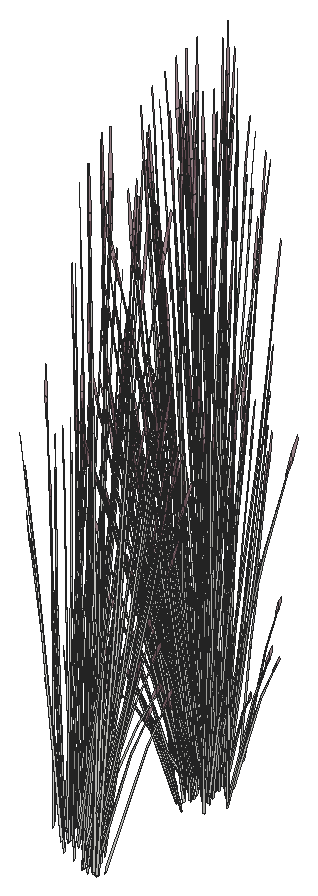
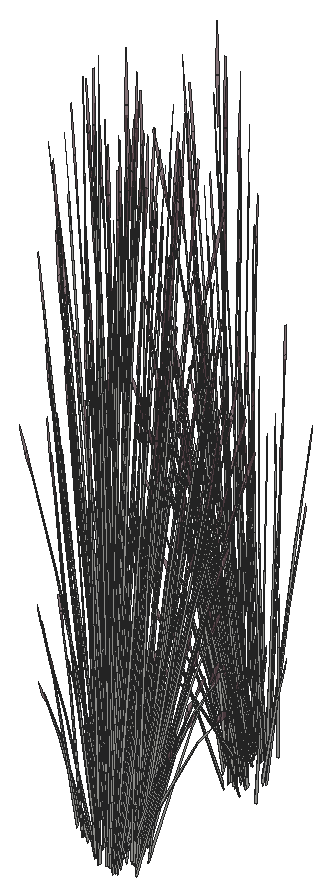
# SketchUp Ruby script. Lengths in inches.
U = 1.inch
M = Sketchup.active_model
def pt(a) = Geom::Point3d.new(a.map { |v| v * U })
def face(e, loops, mat)
  f = e.add_face(loops[0].map { |a| pt(a) })
  loops[1..].each { |l| e.add_face(l.map { |a| pt(a) }).erase! }
  f.material = f.back_material = mat if mat
  f
end
# faces: each face lists its corners as indices into pts; further lists are holes
def faces(e, pts, list, mat = nil) = list.each { |f| face(e, (f[0].is_a?(Array) ? f : [f]).map { |l| l.map { |i| pts[i] } }, mat) }
# xy, xz, yz: faces in a plane at the given z, y or x. An outline is a flat list of corners, or four numbers for a rectangle; further outlines are holes
def ring(l) = l.size == 4 ? [[l[0], l[1]], [l[2], l[1]], [l[2], l[3]], [l[0], l[3]]] : l.each_slice(2).to_a
def flat(e, list, mat, &to3) = list.each { |f| face(e, (f[0].is_a?(Array) ? f : [f]).map { |l| ring(l).map { |u, v| to3.(u, v) } }, mat) }
def xy(e, z, list, mat = nil) = flat(e, list, mat) { |x, y| [x, y, z] }
def xz(e, y, list, mat = nil) = flat(e, list, mat) { |x, z| [x, y, z] }
def yz(e, x, list, mat = nil) = flat(e, list, mat) { |y, z| [x, y, z] }
def lines(e, pts, list) = list.each { |a, b| e.add_line(pt(pts[a]), pt(pts[b])) }
# prism: a flat outline (further loops are holes) pulled along v
def prism(e, loops, v, mat = nil)
  f = face(e, loops, mat); d = Geom::Vector3d.new(v.map { |x| x * U })
  f.pushpull(f.normal.samedirection?(d) ? d.length : -d.length)
end
def box(e, o, s, mat = nil) = prism(e, [[o, [o[0] + s[0], o[1], o[2]], [o[0] + s[0], o[1] + s[1], o[2]], [o[0], o[1] + s[1], o[2]]]], [0, 0, s[2]], mat)
def at(x, y, z, deg = 0) = Geom::Transformation.translation(pt([x, y, z])) * Geom::Transformation.rotation(ORIGIN, Z_AXIS, deg.degrees)
def axes(o, x, y, z) = Geom::Transformation.new([*x, 0, *y, 0, *z, 0, *pt(o).to_a, 1])
def part(name) = M.definitions.add(name)
# library, detail: a bought-in or finely detailed component or shape, given as its bounding box
def library(name, o, s) = part(name).tap { |d| box(d.entities, o, s) }
def detail(e, o, s) = box(e.add_group.entities, o, s)
def put(e, d, t, mat = nil) = e.add_instance(d, t).tap { |i| i.material = mat if mat }
def group(e, t, mat = nil) = e.add_group.tap { |g| g.transformation = t; g.material = mat if mat }.entities
root = M.entities
M.materials.add("LightPink_Translucent").color = [144, 107, 117]
M.materials["LightPink_Translucent"].alpha = 0.75
c1 = part("blade")
p = [[2.15,0.21,22],[0,0.17,0],[0.09,0.45,0],[2.18,0.31,22],[2.29,0.31,22],[0.38,0.45,0],
  [2.48,0.24,33],[2.49,0.24,33],[2.48,0.22,33]]
faces(c1.entities,p,[[0,1,2,3],[4,5,2,3],[6,3,4,7],[8,0,3,6]])
c2 = part("seeds")
p = [[0.3,-0.1,1.38],[-0.01,-0.03,1.59],[-0.01,-0.03,0.03],[0.14,-0.07,-0.07],[0.29,-0.03,3],[0.15,0.01,3.11]]
faces(c2.entities,p,[[0,1,2,3],[1,0,4,5]],"LightPink_Translucent")
c3 = part("blade with seeds")
put(c3.entities,c1,at(0,0,0))
put(c3.entities,c2,axes([2.4,0.25,30.99],[1.5799,-0.05474,1.17369],[-0.12525,1.92788,0.29478],[-0.07173,-0.02425,1.56792]))
put(root,c3,axes([331.53,378.59,1400.62],[0.26075,0.2802,0.1448],[-0.2175,0.31612,-0.41347],[-0.06054,0.04274,1.26744]))
put(root,c3,axes([329.47,378.67,1402.73],[-0.08753,-0.42921,0.48003],[0.34336,-0.07449,0.3958],[-0.1012,0.10094,0.9933]))
put(root,c3,axes([329.41,378.58,1402.73],[-0.2423,-0.19613,0.0643],[0.14107,-0.2793,0.50621],[-0.07768,0.0903,0.77189]))
put(root,c3,axes([329.52,378.07,1401.875],[0.12246,-0.09864,1.71376],[0.1031,0.45582,0.13857],[-0.19225,0.10302,0.73262]))
put(root,c3,axes([332.21,379.08,1402.98],[0.35281,0.01123,-0.71045],[-0.0237,0.47284,0.08574],[0.14947,0.0499,1.00501]))
put(root,c3,axes([331.8125,379.46,1400.48],[0.33032,-0.23318,0.49651],[0.19744,0.41812,0],[-0.07523,0.05311,1.57504]))
put(root,c3,axes([331.34,379.09,1400.29],[0.15345,0.53576,-0.06012],[-0.43845,0.18773,0],[0.00536,0.01871,1.72173]))
put(root,c3,axes([331.51,379.67,1400.03],[-0.32928,-0.11539,-0.30978],[0.08291,-0.40636,0.30978],[-0.06638,0.04686,1.38974]))
put(root,c3,axes([329.14,378.84,1400.59],[0.12266,0.03828,1.43002],[0.07906,0.39104,-0.30754],[-0.16661,0.0732,0.61141]))
put(root,c3,axes([329.6875,378.52,1403.05],[0.30722,-0.06665,0.35414],[0.08112,0.381,-0.4572],[-0.08804,0.10234,0.87481]))
put(root,c3,axes([332.78,378.12,1400.375],[0.44133,0,0],[0,0.52122,-0.51607],[0,0.11871,1.63711]))
put(root,c3,axes([328.5,378.35,1402.71],[0.04504,0.01251,1.77383],[0.13934,0.41205,-0.16761],[-0.0922,0.10815,0.31391]))
put(root,c3,axes([332.61,378.38,1400.2],[-0.44111,-0.00373,-0.04976],[0,-0.52122,0.49943],[-0.01386,0.11865,1.58352]))
put(root,c3,axes([331.65,377.93,1400.67],[0.39748,0.22252,-0.29095],[-0.19139,0.46966,-0.50002],[0.01249,0.11531,1.59708]))
put(root,c3,axes([328.88,379.66,1400.77],[0.14709,-0.21136,1.1486],[0.05804,0.3346,0.84392],[-0.1063,0.05991,0.25299]))
put(root,c3,axes([332.42,379.27,1402.53],[0.20082,0.29199,-0.35414],[-0.2293,0.2764,0.4572],[0.1165,0.04206,0.87481]))
put(root,c3,axes([332.52,378.46,1400.03],[-0.24637,0.29097,-0.30978],[-0.24637,-0.29097,0.30978],[0,0.09372,1.38974]))
put(root,c3,axes([331.46,378.49,1400.67],[0.04113,0.53214,-0.29095],[-0.42835,0.03218,-0.50002],[-0.07543,0.07088,1.59708]))
put(root,c3,axes([332.32,379.38,1402.73],[-0.01777,0.35463,0.0643],[-0.26836,-0.00972,0.50621],[0.1028,0.03711,0.77189]))
put(root,c3,axes([331.61,378.28,1400.21],[-0.17124,0.42022,-0.44739],[-0.35581,-0.20224,0.21531],[0,0.09687,1.43643]))
put(root,c3,axes([329.43,378.75,1402.53],[-0.30722,0.06665,-0.35414],[-0.08112,-0.381,0.4572],[-0.08804,0.10234,0.87481]))
put(root,c3,axes([332.34,379.27,1402.73],[-0.26024,0.30729,0.48003],[-0.22444,-0.32634,0.3958],[0.1221,0.05668,0.9933]))
put(root,c3,axes([328.99,379.6,1403.65],[0.31145,0.12449,-0.06488],[-0.0958,0.38314,-0.29416],[-0.05094,0.05817,0.97024]))
put(root,c3,axes([331.2,378.9,1400.06],[-0.23773,0.35053,-0.62353],[-0.29532,-0.31785,-0.16365],[-0.09526,0.08744,1.37633]))
put(root,c3,axes([331.52,379.625,1403.05],[-0.05451,-0.37564,0.35414],[0.31161,-0.09919,-0.4572],[0.0837,0.10765,0.87481]))
put(root,c3,axes([331.62,379.49,1400.33],[0.44186,0.15158,0.30756],[-0.11054,0.54181,-0.36492],[-0.07313,0.06781,1.64885]))
put(root,c3,axes([331.59,379.85,1400.02],[-0.33032,0.23318,-0.49651],[-0.19744,-0.41812,0],[-0.07523,0.05311,1.57504]))
put(root,c3,axes([332.6875,378.47,1400.02],[0,0.46636,-0.49651],[-0.39487,0,0],[0,0.10622,1.57504]))
put(root,c3,axes([331.7,378.52,1401.875],[-0.1311,-0.08035,1.71376],[0.27131,-0.33708,0.13857],[0.16909,0.15206,0.73262]))
put(root,c3,axes([331.72,377.47,1402.47],[-0.30498,-0.24231,1.38283],[0.32203,-0.37727,0.59665],[0.0984,0.22736,1.33663]))
put(root,c3,axes([329.53,378.49,1403.03],[0.32648,0.25715,-0.1216],[-0.18809,0.3724,-0.67495],[-0.09224,0.12945,1.02557]))
put(root,c3,axes([332.18,379.4375,1400.77],[-0.19872,-0.13409,1.1486],[0.2566,-0.13625,0.84392],[0.06921,0.11541,0.25299]))
put(root,c3,axes([331.49,379.82,1403.03],[0.21031,-0.39918,-0.1216],[0.30457,0.22997,-0.67495],[0.10587,0.11278,1.02557]))
put(root,c3,axes([329.97,378.375,1401.875],[0.08815,-0.14329,1.71376],[0.22258,0.38678,0.13857],[-0.15267,0.17614,0.73262]))
put(root,c3,axes([329.6875,378.79,1402.68],[0.09067,0.42583,-0.51099],[-0.34336,0.07449,-0.3958],[-0.0984,0.11438,0.97773]))
put(root,c3,axes([330.1,379.28,1403.05],[0.23881,-0.24554,0.35414],[0.22606,0.28036,-0.4572],[-0.0344,0.14245,0.87481]))
put(root,c3,axes([331.89,379.78,1400.375],[0.22066,0.46731,0],[-0.36918,0.26061,-0.51607],[-0.08408,0.05936,1.63711]))
put(root,c3,axes([331.21,380.15,1402.71],[0.00104,-0.05646,1.77383],[0.30246,-0.2491,-0.16761],[0.10506,0.08891,0.31391]))
put(root,c3,axes([332.24,379.9375,1399.49],[0.02571,-0.06733,1.76342],[0.32373,-0.19829,-0.26939],[0.09815,0.10263,0.30037]))
put(root,c3,axes([331.7,377.93,1400.84],[-0.00964,-0.43909,1.41272],[0.43635,0.11382,0.59816],[-0.1032,0.24027,1.3335]))
put(root,c3,axes([331.8125,378.41,1400.09],[0.12941,0.42699,-0.69212],[-0.37279,0.15378,-0.18165],[0.0143,0.14459,1.52773]))
put(root,c3,axes([329.88,379.5,1402.73],[-0.29004,-0.02173,0.0643],[0.00795,-0.32812,0.50621],[-0.03035,0.12569,0.77189]))
put(root,c3,axes([329.27,379.88,1399.49],[0.04734,0.04659,1.76342],[0.08027,0.4317,-0.26939],[-0.10492,0.09206,0.30037]))
put(root,c3,axes([329.98,379.53,1402.73],[-0.25132,-0.3182,0.48003],[0.2669,-0.27442,0.3958],[-0.04636,0.14929,0.9933]))
put(root,c3,axes([331.74,379.62,1402.68],[0.34827,-0.11086,-0.51099],[0.06092,0.41983,-0.3958],[0.09354,0.12031,0.97773]))
put(root,c3,axes([330.77,379.6875,1403.05],[0.1064,-0.35863,0.35414],[0.31043,0.1046,-0.4572],[0.02846,0.14439,0.87481]))
put(root,c3,axes([332.22,380.05,1400.67],[-0.22633,-0.01463,1.0506],[0.14947,-0.31064,0.58006],[0.08941,0.11036,0.8241]))
put(root,c3,axes([331.56,379.97,1402.73],[-0.16041,0.29625,0.0643],[-0.22843,-0.17248,0.50621],[0.07385,0.09498,0.77189]))
put(root,c3,axes([331.1875,380.97,1403.65],[0.2439,-0.26754,-0.06488],[0.22348,0.29302,-0.29416],[0.01573,0.08303,0.97024]))
put(root,c3,axes([331.63,379.88,1402.73],[-0.35104,0.10702,0.48003],[-0.06092,-0.41983,0.3958],[0.08256,0.12373,0.9933]))
put(root,c3,axes([329.9,378.73,1401.875],[0.06572,-0.16029,1.71376],[0.27569,0.33172,0.13857],[-0.12437,0.20675,0.73262]))
put(root,c3,axes([331.48,379.3,1400.59],[0.00623,-0.15459,1.43002],[0.29764,-0.17268,-0.30754],[0.09188,0.18503,0.61141]))
put(root,c3,axes([330.67,380.01,1402.73],[-0.26007,0.1585,0.0643],[-0.12729,-0.28902,0.50621],[0.02512,0.1274,0.77189]))
put(root,c3,axes([329.98,379.63,1402.53],[-0.23881,0.24554,-0.35414],[-0.22606,-0.28036,0.4572],[-0.0344,0.14245,0.87481]))
put(root,c3,axes([329.15,379.56,1402.72],[-0.00877,0.09229,1.74944],[0.24897,0.32105,-0.27667],[-0.06518,0.15182,0.14031]))
put(root,c3,axes([329.95,379.35,1403.4],[0.3879,0.02311,-0.13498],[-0.0106,0.43749,-0.74919],[-0.02694,0.1685,1.13838]))
put(root,c3,axes([330.67,379.84,1403.03],[0.34538,-0.21713,-0.1216],[0.16972,0.38536,-0.67495],[0.04557,0.16239,1.02557]))
put(root,c3,axes([330.77,379.98,1403.0625],[-0.34777,-0.12192,0.53283],[0.11892,-0.40083,0.43934],[0.0209,0.15763,1.10256]))
put(root,c3,axes([330.13,380.58,1400.77],[-0.00913,-0.2773,1.1486],[0.22824,0.19778,0.84392],[-0.04489,0.13217,0.25299]))
put(root,c3,axes([330.73,379.92,1399.49],[0.05712,-0.02538,1.76342],[0.34359,0.13968,-0.26939],[0.01005,0.15742,0.30037]))
put(root,c3,axes([330.21,379.51,1403],[0.25266,0.31335,-0.5672],[-0.2669,0.27442,-0.43934],[-0.03844,0.15921,1.08528]))
put(root,c3,axes([329.9375,379.98,1400.82],[0.32063,-0.08258,0.06507],[0.07371,0.33271,-0.86304],[-0.02033,0.16842,0.7736]))
put(root,c3,axes([330.96,379.82,1402.68],[0.34695,0.11691,-0.51099],[-0.11892,0.40083,-0.3958],[0.03181,0.16138,0.97773]))
put(root,c3,axes([331.16,378.99,1401.875],[-0.08068,-0.14973,1.71376],[0.3728,-0.12606,0.13857],[0.08426,0.23506,0.73262]))
put(root,c3,axes([330.8,380.0625,1402.53],[-0.1064,0.35863,-0.35414],[-0.31043,-0.1046,0.4572],[0.02846,0.14439,0.87481]))
put(root,c3,axes([330.13,379.37,1403.34],[-0.00918,0.43138,-0.7886],[-0.38672,-0.02897,0.09517],[-0.04081,0.18275,1.11556]))
put(root,c3,axes([329.125,380.5,1402.71],[0.04004,-0.02816,1.77383],[0.33095,0.18728,-0.16761],[-0.00778,0.15594,0.31391]))
put(root,c3,axes([330.5,379.06,1401.875],[-0.00864,-0.17899,1.71376],[0.37441,0.11874,0.13857],[-0.02316,0.25508,0.73262]))
put(root,c3,axes([330.84,379.74,1402.98],[0.16845,0.3792,-0.71045],[-0.34676,0.21133,0.08574],[0.03939,0.18322,1.00501]))
put(root,c3,axes([329.86,380.34,1400.59],[0.11138,-0.07357,1.43002],[0.27499,0.22183,-0.30754],[-0.08185,0.19194,0.61141]))
put(root,c3,axes([330.58,380.7,1402.72],[0.04474,0.0751,1.74944],[0.36104,0.0295,-0.27667],[0.03631,0.16562,0.14031]))
put(root,c3,axes([330.01,379.98,1401.36],[0.00775,-0.24075,1.54345],[0.34877,0.12716,0.21329],[-0.03022,0.25658,0.72882]))
put(root,c3,axes([330.27,391.54,1401.875],[0.08068,0.14973,1.71376],[-0.3728,0.12606,0.13857],[-0.08426,-0.23506,0.73262]))
put(root,c3,axes([330.89,390.55,1402.72],[-0.05398,-0.06539,1.74944],[-0.36026,0.04145,-0.27667],[-0.0575,-0.15639,0.14031]))
put(root,c3,axes([331.72,391.33,1400.59],[-0.10032,0.0944,1.43002],[-0.30046,-0.16522,-0.30754],[0.05569,-0.20547,0.61141]))
put(root,c3,axes([331.27,391.66,1402.98],[-0.16845,-0.3792,-0.71045],[0.34676,-0.21133,0.08574],[-0.03939,-0.18322,1.00501]))
put(root,c3,axes([330.17,391.15,1400.59],[-0.02137,0.15256,1.43002],[-0.31245,0.12771,-0.30754],[-0.07303,-0.19719,0.61141]))
put(root,c3,axes([330.98,390.81,1399.49],[-0.0592,0.0168,1.76342],[-0.32738,-0.18913,-0.26939],[0.00549,-0.15776,0.30037]))
put(root,c3,axes([331.97,392.03,1402.98],[0.00918,-0.43138,-0.71045],[0.38672,0.02897,0.08574],[0.04081,-0.18275,1.00501]))
put(root,c3,axes([332.51,391.35,1402.72],[-0.00341,-0.09282,1.74944],[-0.28775,-0.26825,-0.27667],[0.04449,-0.16261,0.14031]))
put(root,c3,axes([331.3,391.33,1402.53],[0.1064,-0.35863,-0.35414],[0.31043,0.1046,0.4572],[-0.02846,-0.14439,0.87481]))
put(root,c3,axes([331.53,391.81,1401.875],[-0.06572,0.16029,1.71376],[-0.27569,-0.33172,0.13857],[0.12437,-0.20675,0.73262]))
put(root,c3,axes([332.43,391.02,1402.71],[-0.03584,0.03562,1.77383],[-0.35118,-0.12018,-0.16761],[-0.01271,-0.15545,0.31391]))
put(root,c3,axes([331.14,391.58,1402.68],[-0.34695,-0.11691,-0.51099],[0.11892,-0.40083,-0.3958],[-0.03181,-0.16138,0.97773]))
put(root,c3,axes([331.35,390.58,1400.77],[0.04528,0.27194,1.1486],[-0.25117,-0.15062,0.84392],[0.02703,-0.13924,0.25299]))
put(root,c3,axes([331.89,391.88,1402.68],[-0.25266,-0.31335,-0.51099],[0.2669,-0.27442,-0.3958],[0.03844,-0.15921,0.97773]))
put(root,c3,axes([330.52,390.34,1402.71],[-0.00658,0.0559,1.77383],[-0.32474,0.20287,-0.16761],[-0.09556,-0.1037,0.31391]))
put(root,c3,axes([330.45,391.33,1403.09],[0.39316,-0.11987,0.53763],[0.06823,0.47021,0.4433],[-0.09247,-0.13858,1.11249]))
put(root,c3,axes([331.34,391.42,1402.73],[0.34777,0.12192,0.48003],[-0.11892,0.40083,0.3958],[-0.0209,-0.15763,0.9933]))
put(root,c3,axes([331.4375,391.5625,1403.03],[-0.34538,0.21713,-0.1216],[-0.16972,-0.38536,-0.67495],[-0.04557,-0.16239,1.02557]))
put(root,c3,axes([332.15,392.05,1403.03],[-0.3879,-0.02311,-0.1216],[0.0106,-0.43749,-0.67495],[0.02694,-0.1685,1.02557]))
put(root,c3,axes([332.13,391.77,1402.53],[0.23881,-0.24554,-0.35414],[0.22606,0.28036,0.4572],[0.0344,-0.14245,0.87481]))
put(root,c3,axes([330.0625,390.9,1400.77],[0.18411,0.16231,1.1486],[-0.26813,0.09757,0.84392],[-0.05737,-0.12474,0.25299]))
put(root,c3,axes([331.43,391.39,1402.73],[0.26007,-0.1585,0.0643],[0.12729,0.28902,0.50621],[-0.02512,-0.1274,0.77189]))
put(root,c3,axes([330.51,391.76,1402.98],[-0.30095,-0.22541,-0.71045],[0.21388,-0.395,0.08574],[-0.10904,-0.13459,1.00501]))
put(root,c3,axes([330.4,391.47,1402.53],[-0.05451,-0.37564,-0.35414],[0.31161,-0.09919,0.4572],[-0.0837,-0.10765,0.87481]))
put(root,c3,axes([330.54,391.43,1402.73],[0.16041,-0.29625,0.0643],[0.22843,0.17248,0.50621],[-0.07385,-0.09498,0.77189]))
put(root,c3,axes([329.92,391.39,1399.49],[-0.03419,0.06144,1.76342],[-0.3455,0.13246,-0.26939],[-0.08346,-0.12049,0.30037]))
put(root,c3,axes([330.49,393.08,1400.1],[-0.14494,-0.47823,-0.69835],[0.41752,-0.17223,-0.18329],[-0.01602,-0.16194,1.54149]))
put(root,c3,axes([329.73,392.01,1401.875],[0.1311,0.08035,1.71376],[-0.27131,0.33708,0.13857],[-0.16909,-0.15206,0.73262]))
put(root,c3,axes([332.43,391.62,1399.49],[-0.05283,-0.03674,1.76342],[-0.13569,-0.41045,-0.26939],[0.09154,-0.11138,0.30037]))
put(root,c3,axes([331.33,391.71,1403.05],[-0.1064,0.35863,0.35414],[-0.31043,-0.1046,-0.4572],[-0.02846,-0.14439,0.87481]))
put(root,c3,axes([330.37,391.77,1402.68],[-0.34827,0.11086,-0.51099],[-0.06092,-0.41983,-0.3958],[-0.09354,-0.12031,0.97773]))
put(root,c3,axes([332.125,391.86,1402.73],[0.25132,0.3182,0.48003],[-0.2669,0.27442,0.3958],[0.04636,-0.14929,0.9933]))
put(root,c3,axes([330.61,391.4,1403.43],[-0.23555,0.44708,-0.13619],[-0.34112,-0.25757,-0.75594],[-0.11858,-0.12631,1.14864]))
put(root,c3,axes([332.22,391.89,1402.73],[0.29004,0.02173,0.0643],[-0.00795,0.32812,0.50621],[0.03035,-0.12569,0.77189]))
put(root,c3,axes([332,392.12,1403.05],[-0.23881,0.24554,0.35414],[-0.22606,-0.28036,-0.4572],[0.0344,-0.14245,0.87481]))
put(root,c3,axes([332.42,392.78,1402.98],[0.18436,-0.36797,-0.71045],[0.32306,0.26151,0.08574],[0.11008,-0.13332,1.00501]))
put(root,c3,axes([330.43,391.71,1400.375],[-0.22066,-0.46731,0],[0.36918,-0.26061,-0.51607],[0.08408,-0.05936,1.63711]))
put(root,c3,axes([332.41,392.6,1402.68],[-0.09067,-0.42583,-0.51099],[0.34336,-0.07449,-0.3958],[0.0984,-0.11438,0.97773]))
put(root,c3,axes([330.92,391.14,1400.13],[-0.2439,0.26754,-0.03893],[-0.22348,-0.29302,-0.17649],[-0.01573,-0.08303,0.58215]))
put(root,c3,axes([329.71,391.27,1402.72],[-0.07594,-0.00329,1.74944],[-0.24177,0.32918,-0.27667],[-0.129,-0.06726,0.14031]))
put(root,c3,axes([332.58,392.91,1403.03],[-0.32648,-0.25715,-0.1216],[0.18809,-0.3724,-0.67495],[0.09224,-0.12945,1.02557]))
put(root,c3,axes([331.23,394.3125,1401.33],[0.305,0.18805,1.51261],[-0.29879,0.40513,0.59816],[-0.13384,-0.24012,1.26806]))
put(root,c3,axes([330.59,391.77,1403.05],[0.05451,0.37564,0.35414],[-0.31161,0.09919,-0.4572],[-0.0837,-0.10765,0.87481]))
put(root,c3,axes([329.63,393.01,1400.02],[0,-0.46636,-0.49651],[0.39487,0,0],[0,-0.10622,1.57504]))
put(root,c3,axes([330.73,391.63,1400.02],[0.33032,-0.23318,-0.49651],[0.19744,0.41812,0],[0.07523,-0.05311,1.57504]))
put(root,c3,axes([332.69,392.4375,1400.59],[-0.12609,-0.01381,1.43002],[-0.12917,-0.37055,-0.30754],[0.1549,-0.10482,0.61141]))
put(root,c3,axes([329.65,392.02,1403.09],[0.29147,-0.34417,0.53763],[0.25138,0.3655,0.4433],[-0.13675,-0.06349,1.11249]))
put(root,c3,axes([333.38,392.8,1402.71],[-0.0461,-0.00354,1.77383],[-0.19143,-0.37951,-0.16761],[0.07688,-0.12478,0.31391]))
put(root,c3,axes([331.12,392.59,1400.06],[0.23773,-0.35053,-0.62353],[0.29532,0.31785,-0.16365],[0.09526,-0.08744,1.37633]))
put(root,c3,axes([332.84,391.76,1400.77],[-0.11756,0.2374,1.1486],[-0.10105,-0.31895,0.84392],[0.09709,-0.07992,0.25299]))
put(root,c3,axes([332.67,392.65,1402.53],[0.30722,-0.06665,-0.35414],[0.08112,0.381,0.4572],[0.08804,-0.10234,0.87481]))
put(root,c3,axes([329.78,392.01,1402.73],[0.01777,-0.35463,0.0643],[0.26836,0.00972,0.50621],[-0.1028,-0.03711,0.77189]))
put(root,c3,axes([330.71,393.2,1400.21],[0.17124,-0.42022,-0.44739],[0.35581,0.20224,0.21531],[0,-0.09687,1.43643]))
put(root,c3,axes([329.68,392.125,1402.53],[-0.20082,-0.29199,-0.35414],[0.2293,-0.2764,0.4572],[-0.1165,-0.04206,0.87481]))
put(root,c3,axes([330.86,393,1400.67],[-0.04113,-0.53214,-0.29095],[0.42835,-0.03218,-0.50002],[0.07543,-0.07088,1.59708]))
put(root,c3,axes([329.8,393.02,1400.03],[0.24637,-0.29097,-0.30978],[0.24637,0.29097,0.30978],[0,-0.09372,1.38974]))
put(root,c3,axes([329.7,391.63,1400.13],[-0.10181,0.3808,-0.03893],[-0.31336,-0.11714,-0.17649],[-0.04758,-0.06228,0.58215]))
put(root,c3,axes([332.42,392.875,1403.05],[-0.30722,0.06665,0.35414],[-0.08112,-0.381,-0.4572],[0.08804,-0.10234,0.87481]))
put(root,c3,axes([330.67,393.55,1400.67],[-0.39748,-0.22252,-0.29095],[0.19139,-0.46966,-0.50002],[-0.01249,-0.11531,1.59708]))
put(root,c3,axes([329.53,393.37,1400.375],[-0.44133,0,0],[0,-0.52122,-0.51607],[0,-0.11871,1.63711]))
put(root,c3,axes([329.61,392.4375,1400.59],[0.06891,0.12984,1.43002],[-0.15879,0.35293,-0.30754],[-0.16304,-0.08436,0.61141]))
put(root,c3,axes([330.81,391.82,1400.03],[0.32928,0.11539,-0.30978],[-0.08291,0.40636,0.30978],[0.06638,-0.04686,1.38974]))
put(root,c3,axes([329.89,392.32,1402.98],[-0.35281,-0.01123,-0.71045],[0.0237,-0.47284,0.08574],[-0.14947,-0.0499,1.00501]))
put(root,c3,axes([332.7,392.8125,1402.73],[0.2423,0.19613,0.0643],[-0.14107,0.2793,0.50621],[0.07768,-0.0903,0.77189]))
put(root,c3,axes([332.63,392.73,1402.73],[0.08753,0.42921,0.48003],[-0.34336,0.07449,0.3958],[0.1012,-0.10094,0.9933]))
put(root,c3,axes([333.55,393.25,1402.72],[0.04898,-0.07104,1.74944],[-0.06269,-0.43574,-0.27667],[0.12289,-0.08262,0.14031]))
put(root,c3,axes([329.875,393.23,1400.33],[-0.32829,0.39208,0.30756],[-0.32849,-0.38796,-0.36492],[-0.01146,-0.11134,1.64885]))
put(root,c3,axes([329.42,391.55,1402.71],[0.02617,0.04654,1.77383],[-0.12614,0.41836,-0.16761],[-0.12775,0.00303,0.31391]))
put(root,c3,axes([330.92,393.41,1400.43],[0.39767,0.22603,0.24065],[-0.19139,0.46966,0.50002],[0,-0.10827,1.60543]))
put(root,c3,axes([330.77,394.05,1400.4375],[0.09355,-0.55261,-0.23429],[0.44354,0.09633,0.51271],[-0.0775,-0.07631,1.5644]))
put(root,c3,axes([329.78,392.42,1402.68],[-0.25628,0.30892,-0.51099],[-0.22444,-0.32634,-0.3958],[-0.13021,-0.047,0.97773]))
put(root,c3,axes([329.97,392.28,1403.05],[0.20082,0.29199,0.35414],[-0.2293,0.2764,-0.4572],[-0.1165,-0.04206,0.87481]))
put(root,c3,axes([329.2,392.83,1400.77],[0.22533,-0.03337,1.1486],[-0.14293,0.29403,0.84392],[-0.11135,-0.04411,0.25299]))
put(root,c3,axes([330.79,393.1,1400.72],[-0.38326,0.02879,0.44739],[-0.03466,-0.47788,-0.21531],[0.06861,-0.04843,1.43643]))
put(root,c3,axes([329.91,392.09,1403.03],[-0.0189,0.47427,-0.1216],[-0.35781,-0.01296,-0.67495],[-0.13781,-0.03295,1.02557]))
put(root,c3,axes([329.8,393.45,1400.48],[0,0.46636,0.49651],[-0.39487,0,0],[0,-0.10622,1.57504]))
put(root,c3,axes([332.59,393.91,1403.03],[-0.17758,-0.42229,-0.1216],[0.31518,-0.20752,-0.67495],[0.13282,-0.05572,1.02557]))
put(root,c3,axes([332.57,393.55,1402.68],[0.09562,-0.42421,-0.51099],[0.32782,0.1454,-0.3958],[0.13199,-0.0389,0.97773]))
put(root,c3,axes([332.06,391.82,1400.375],[0.22066,-0.46731,0],[0.36918,0.26061,-0.51607],[0.08408,0.05936,1.63711]))
put(root,c3,axes([329.46,392.75,1401.875],[0.14639,-0.01056,1.71376],[-0.09712,0.45778,0.13857],[-0.20862,-0.02831,0.73262]))
put(root,c3,axes([330.73,393.82,1400.21],[-0.21202,-0.39143,-0.44739],[0.32115,-0.27564,0.21531],[-0.06861,-0.04843,1.43643]))
put(root,c3,axes([330.78,393.27,1400.36],[0.15345,0.52148,0.45755],[-0.43845,0.18134,0.17955],[0.00536,-0.09582,1.58856]))
put(root,c3,axes([332.92,393.67,1399.98],[-0.22732,0.05597,1.41583],[-0.03618,-0.44548,0.08104],[0.15921,-0.06743,0.80566]))
put(root,c3,axes([333.34,393.28,1400.26],[-0.21881,-0.29821,-0.06488],[0.23965,-0.27324,-0.29416],[0.0679,-0.01924,0.97024]))
put(root,c3,axes([330.7,393.68,1400.72],[-0.17124,0.42022,0.44739],[-0.35581,-0.20224,-0.21531],[0,-0.09687,1.43643]))
put(root,c3,axes([331.33,393.3125,1400.21],[0,-0.53961,0],[0.44133,0,0],[0,0,1.79456]))
put(root,c3,axes([331.87,392.07,1400.48],[-0.33032,-0.23318,0.49651],[0.19744,-0.41812,0],[0.07523,0.05311,1.57504]))
put(root,c3,axes([332.51,393.7,1402.98],[0.31014,-0.20596,-0.71045],[0.17284,0.42397,0.08574],[0.14985,-0.04816,1.00501]))
put(root,c3,axes([330.54,393.97,1400.06],[-0.36714,-0.07646,-0.62353],[0.07747,-0.47163,-0.16365],[-0.10956,-0.05715,1.37633]))
put(root,c3,axes([331.12,392.97,1400.36],[-0.29264,0.42323,0.45755],[-0.34767,-0.3736,0.17955],[0.07055,-0.04224,1.58856]))
put(root,c3,axes([331.44,393.73,1400.3],[-0.32829,-0.4014,-0.06131],[0.32849,-0.40164,0],[-0.01146,-0.01402,1.75571]))
put(root,c3,axes([330.61,392.28,1400.47],[-0.10196,0.46348,0.17642],[-0.3731,-0.13116,0.35086],[0.06445,-0.00226,1.60407]))
put(root,c3,axes([332.47,393.79,1403.05],[-0.29332,-0.1301,0.35414],[0.08555,-0.37955,-0.4572],[0.11809,-0.0348,0.87481]))
put(root,c3,axes([329.4,393.09,1402.73],[0.09971,-0.42522,0.48003],[0.32782,0.1454,0.3958],[-0.12892,0.02555,0.9933]))
put(root,c3,axes([330.46,392.65,1399.59],[-0.3474,0.18671,1.28929],[-0.11057,-0.53572,0.50096],[0.21332,0.00891,1.46642]))
put(root,c3,axes([331.39,392.79,1400.62],[0.06809,-0.4162,0.1448],[0.33266,0.07225,-0.41347],[0.06054,0.04274,1.26744]))
put(root,c3,axes([329.37,392.98,1402.73],[-0.12963,-0.31798,0.0643],[0.23638,-0.15564,0.50621],[-0.1042,0.03071,0.77189]))
put(root,c3,axes([330.82,393.78,1400.36],[0.44609,0.09826,0.45755],[-0.09078,0.55493,0.17955],[-0.06519,-0.05359,1.58856]))
put(root,c3,axes([333.17,393.38,1399.49],[-0.01845,-0.0708,1.76342],[0.12793,-0.41416,-0.26939],[0.12905,-0.00596,0.30037]))
put(root,c3,axes([329.36,393.31,1399.49],[0.00895,0.0735,1.76342],[-0.18044,0.38382,-0.26939],[-0.12817,-0.01935,0.30037]))
put(root,c3,axes([331.25,392.9,1400.72],[-0.21202,-0.39143,0.44739],[0.32115,-0.27564,-0.21531],[0.06861,0.04843,1.43643]))
put(root,c3,axes([330.15,394.69,1400.03],[-0.08291,-0.40636,-0.30978],[0.32928,-0.11539,0.30978],[-0.06638,-0.04686,1.38974]))
put(root,c3,axes([330.58,394.67,1400.47],[0.37926,-0.12378,0.17642],[0.09365,0.46065,0.35086],[-0.03382,-0.06712,1.60407]))
put(root,c3,axes([331.36,392.93,1400.67],[0.35635,-0.30962,-0.29095],[0.23697,0.43749,-0.50002],[0.08792,0.04443,1.59708]))
put(root,c3,axes([332.78,393.74,1402.53],[0.29332,0.1301,-0.35414],[-0.08555,0.37955,0.4572],[0.11809,-0.0348,0.87481]))
put(root,c3,axes([330.0625,394.87,1400.02],[-0.33032,-0.23318,-0.49651],[0.19744,-0.41812,0],[-0.07523,-0.05311,1.57504]))
put(root,c3,axes([332.26,392.1,1400.02],[0.33032,0.23318,-0.49651],[-0.19744,0.41812,0],[0.07523,0.05311,1.57504]))
put(root,c3,axes([329.33,393.14,1402.53],[-0.29332,-0.1301,-0.35414],[0.08555,-0.37955,0.4572],[-0.11809,0.0348,0.87481]))
put(root,c3,axes([331.63,393.43,1400.21],[0.39487,0,0],[0,0.48281,0],[0,0,1.78407]))
put(root,c3,axes([330.96,394.04,1400.67],[-0.35635,0.30962,-0.29095],[-0.23697,-0.43749,-0.50002],[-0.08792,-0.04443,1.59708]))
put(root,c3,axes([331.74,392.3,1400.47],[-0.37926,0.12378,0.17642],[-0.09365,-0.46065,0.35086],[0.03382,0.06712,1.60407]))
put(root,c3,axes([331.98,393.27,1401.875],[-0.14639,0.01056,1.71376],[0.09712,-0.45778,0.13857],[0.20862,0.02831,0.73262]))
put(root,c3,axes([332.17,392.28,1400.03],[0.08291,0.40636,-0.30978],[-0.32928,0.11539,0.30978],[0.06638,0.04686,1.38974]))
put(root,c3,axes([332.73,393.9,1402.73],[0.12963,0.31798,0.0643],[-0.23638,0.15564,0.50621],[0.1042,-0.03071,0.77189]))
put(root,c3,axes([331.5,393.1875,1400.38],[-0.44609,-0.09826,0.49198],[0.09078,-0.55493,0.19306],[0.06519,0.05359,1.70813]))
put(root,c3,axes([332.71,393.79,1402.73],[-0.09971,0.42522,0.48003],[-0.32782,-0.1454,0.3958],[0.12892,-0.02555,0.9933]))
put(root,c3,axes([331.15,394.56,1400.2],[-0.11516,-0.40207,0],[0.32884,-0.1408,0],[0,0,1.54371]))
put(root,c3,axes([330.93,394.18,1400.62],[-0.06809,0.4162,0.1448],[-0.33266,-0.07225,-0.41347],[-0.06054,-0.04274,1.26744]))
put(root,c3,axes([329.64,393.1,1403.05],[0.29332,0.1301,0.35414],[-0.08555,0.37955,-0.4572],[-0.11809,0.0348,0.87481]))
put(root,c3,axes([331.58,394.5,1400.18],[0.37054,-0.15823,-0.19198],[0.1302,0.45581,0.00008],[0.0409,-0.01749,1.73897]))
put(root,c3,axes([331.71,394.69,1400.47],[0.10196,-0.46348,0.17642],[0.3731,0.13116,0.35086],[-0.06445,0.00226,1.60407]))
put(root,c3,axes([331.62,393.64,1400.21],[0.24637,0.30123,0],[-0.24637,0.30123,0],[0,0,1.69266]))
put(root,c3,axes([330.22,393.08,1401.34],[0.10032,-0.06746,1.77064],[0.0346,0.47103,0.13857],[-0.2173,0.0625,0.63284]))
put(root,c3,axes([332.29,393.51,1400.47],[-0.2773,-0.3397,0.17642],[0.27945,-0.32949,0.35086],[-0.03063,0.06937,1.60407]))
put(root,c3,axes([331.78,393,1400.06],[0.36714,0.07646,-0.62353],[-0.07747,0.47163,-0.16365],[0.10956,0.05715,1.37633]))
put(root,c3,axes([333.4,393.82,1400.77],[-0.21807,0.07699,1.1486],[0.10265,-0.31819,0.84392],[0.11568,0.02177,0.25299]))
put(root,c3,axes([331.07,394.74,1400.2],[-0.35581,-0.20937,0],[0.17124,-0.43505,0],[0,0,1.62707]))
put(root,c3,axes([331.36,394.18,1400.46],[-0.34464,-0.37536,-0.25192],[0.29,-0.42149,0.5513],[-0.0928,0.04391,1.68216]))
put(root,c3,axes([330.45,394.9,1400.48],[0.33032,0.23318,0.49651],[-0.19744,0.41812,0],[-0.07523,-0.05311,1.57504]))
put(root,c3,axes([331.62,393.29,1400.72],[0.17124,-0.42022,0.44739],[0.35581,0.20224,-0.21531],[0,0.09687,1.43643]))
put(root,c3,axes([333.3,395.17,1402.71],[-0.03191,-0.04083,1.77383],[0.06981,-0.43764,-0.16761],[0.12571,-0.02796,0.31391]))
put(root,c3,axes([329.14,393.39,1402.72],[-0.05763,0.06055,1.74944],[0.0049,0.44239,-0.27667],[-0.13211,0.05753,0.14031]))
put(root,c3,axes([331.55,393.53,1400.29],[0,0.53934,-0.05637],[-0.44133,0,0],[0,0.01695,1.79368]))
put(root,c3,axes([329.53,393.33,1402.68],[-0.09562,0.42421,-0.51099],[-0.32782,-0.1454,-0.3958],[-0.13199,0.0389,0.97773]))
put(root,c3,axes([329.51,392.97,1403.03],[0.17758,0.42229,-0.1216],[-0.31518,0.20752,-0.67495],[-0.13282,0.05572,1.02557]))
put(root,c3,axes([331.58,393.15,1400.21],[0.21202,0.39143,-0.44739],[-0.32115,0.27564,0.21531],[0.06861,0.04843,1.43643]))
put(root,c3,axes([333.02,394.8,1401.93],[-0.06755,-0.39203,-0.03492],[0.31928,-0.09013,-0.15832],[0.06667,0.02485,0.52218]))
put(root,c3,axes([330.26,395.15,1400.375],[-0.22066,0.46731,0],[-0.36918,-0.26061,-0.51607],[-0.08408,-0.05936,1.63711]))
